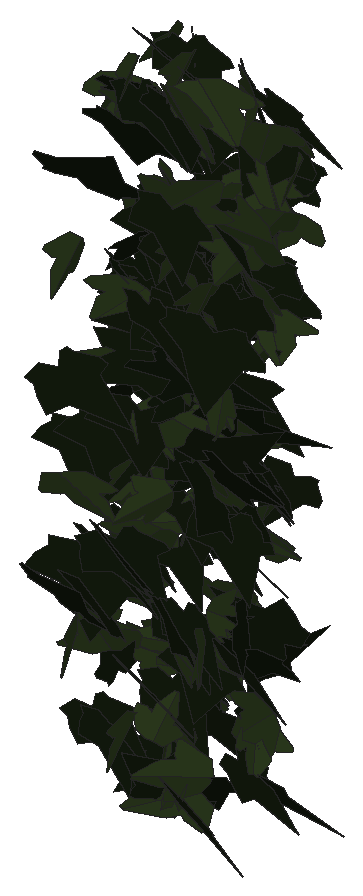
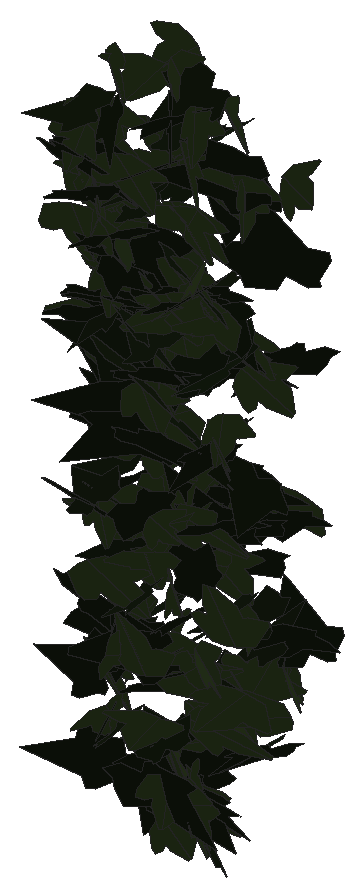
# SketchUp Ruby script. Lengths in millimetres.
U = 1.mm
M = Sketchup.active_model
def pt(a) = Geom::Point3d.new(a.map { |v| v * U })
def face(e, loops, mat)
  f = e.add_face(loops[0].map { |a| pt(a) })
  loops[1..].each { |l| e.add_face(l.map { |a| pt(a) }).erase! }
  f.material = f.back_material = mat if mat
  f
end
# faces: each face lists its corners as indices into pts; further lists are holes
def faces(e, pts, list, mat = nil) = list.each { |f| face(e, (f[0].is_a?(Array) ? f : [f]).map { |l| l.map { |i| pts[i] } }, mat) }
# xy, xz, yz: faces in a plane at the given z, y or x. An outline is a flat list of corners, or four numbers for a rectangle; further outlines are holes
def ring(l) = l.size == 4 ? [[l[0], l[1]], [l[2], l[1]], [l[2], l[3]], [l[0], l[3]]] : l.each_slice(2).to_a
def flat(e, list, mat, &to3) = list.each { |f| face(e, (f[0].is_a?(Array) ? f : [f]).map { |l| ring(l).map { |u, v| to3.(u, v) } }, mat) }
def xy(e, z, list, mat = nil) = flat(e, list, mat) { |x, y| [x, y, z] }
def xz(e, y, list, mat = nil) = flat(e, list, mat) { |x, z| [x, y, z] }
def yz(e, x, list, mat = nil) = flat(e, list, mat) { |y, z| [x, y, z] }
def lines(e, pts, list) = list.each { |a, b| e.add_line(pt(pts[a]), pt(pts[b])) }
# prism: a flat outline (further loops are holes) pulled along v
def prism(e, loops, v, mat = nil)
  f = face(e, loops, mat); d = Geom::Vector3d.new(v.map { |x| x * U })
  f.pushpull(f.normal.samedirection?(d) ? d.length : -d.length)
end
def box(e, o, s, mat = nil) = prism(e, [[o, [o[0] + s[0], o[1], o[2]], [o[0] + s[0], o[1] + s[1], o[2]], [o[0], o[1] + s[1], o[2]]]], [0, 0, s[2]], mat)
def at(x, y, z, deg = 0) = Geom::Transformation.translation(pt([x, y, z])) * Geom::Transformation.rotation(ORIGIN, Z_AXIS, deg.degrees)
def axes(o, x, y, z) = Geom::Transformation.new([*x, 0, *y, 0, *z, 0, *pt(o).to_a, 1])
def part(name) = M.definitions.add(name)
# library, detail: a bought-in or finely detailed component or shape, given as its bounding box
def library(name, o, s) = part(name).tap { |d| box(d.entities, o, s) }
def detail(e, o, s) = box(e.add_group.entities, o, s)
def put(e, d, t, mat = nil) = e.add_instance(d, t).tap { |i| i.material = mat if mat }
def group(e, t, mat = nil) = e.add_group.tap { |g| g.transformation = t; g.material = mat if mat }.entities
root = M.entities
M.materials.add("efeu1").color = [18, 25, 13]
M.materials.add("efeu2").color = [43, 57, 29]
c1 = part("ivyleaf_10")
p = [[0,12.8,-0.8],[-1.5,51.3,-10.9],[-4.9,51,-11.6],[-13.6,26.5,-7.3],[-13.2,15.9,-4.6],[-21.1,19.3,-7.2],
  [-29.5,16.3,-8.3],[-29.2,8.3,-6.2],[-19.7,-9.8,0.5],[-7.6,-13,4],[1,-12.2,5.8],[-0.4,51.1,-11.1],
  [-1.5,51.1,-10.9],[1,-12.4,5.9],[16.9,-12.4,3.5],[35.1,9.1,-5.1],[35,12.9,-6.1],[20.5,16.4,-4.9],
  [15.8,15,-3.8],[15.3,27.6,-7.1],[12.8,31.3,-7.8]]
faces(c1.entities,p,[[0,1,2,3,4,5,6,7,8,9,10],[11,12,0,13,14,15,16,17,18,19,20]],"efeu2")
c2 = part("ivyleaf_9")
p = [[39.1,54.8,31.7],[34.5,51.8,30.2],[-5.3,25.2,17.3],[-17.9,28.3,20.9],[-21.6,21.7,17],[-20.2,4.3,5.3],
  [-22.9,-0.3,2.5],[-17.1,-4,-0.6],[-2,-2.1,-1.2],[-0.7,-15.4,-10.1],[16.6,-22.3,-16.7],[21.1,-15.1,-12.5],
  [32.7,-10.7,-11],[46.1,-1.8,-6.6],[30.8,11.2,3.8]]
faces(c2.entities,p,[[0,1,2,3,4,5,6,7,8,9,10,11,12,13,14]],"efeu1")
put(root,c1,axes([3456.2,839,2506.2],[-0.05855,-0.88523,-0.54951],[0.0878,0.54805,-0.88546],[1.98103,-0.05046,0.023]))
put(root,c2,axes([3449.5,796,2071.7],[-1.0325,-0.74393,-0.21149],[0.2375,0.17075,-0.92073],[1.45265,-0.55668,0.00021]))
put(root,c2,axes([3430.4,804.6,2397.7],[2.21147,0.04712,0.13204],[-0.2513,-0.00281,1.16293],[0.08971,-1.16945,0.00252]))
put(root,c2,axes([3458.7,818.3,2121.9],[0.6766,0.85856,0.21497],[0.18074,0.19332,-0.92916],[-1.67473,0.36773,-0.01343]))
put(root,c2,axes([3437.2,751.5,1880],[1.88054,-0.38188,-0.22943],[0.43927,-0.03862,1.05832],[-0.72521,-1.01364,0.04611]))
put(root,c1,axes([3453.5,863.1,1856.2],[-1.35623,-0.42287,-0.54351],[0.92299,0.24712,-0.82811],[0.93049,-0.86148,0.02925]))
put(root,c1,axes([3459,756.6,1842.1],[0.63988,-0.87304,0.59235],[0.57146,-0.51681,-0.93213],[1.92488,0.44365,0.07982]))
put(root,c1,axes([3442.7,808.3,1816.7],[0.3833,0.20067,0.88907],[0.9971,0.71958,-0.28109],[-1.41943,0.55966,0.04263]))
put(root,c1,axes([3454.9,870.4,1948.7],[-1.6766,-0.05765,0.45851],[0.87841,-0.0604,0.87917],[-0.04398,0.99128,0.08024]))
put(root,c1,axes([3462.5,824.9,1937.6],[-0.86012,0.77193,-0.35043],[0.29869,-0.31406,-0.89423],[-1.58554,-0.47792,0.02164]))
put(root,c1,axes([3468.9,865.7,2211.1],[-0.46907,-0.9224,-0.17623],[0.40552,0.12251,-0.93926],[1.74064,-0.27711,0.17133]))
put(root,c2,axes([3465.7,788.7,1914.7],[-1.45807,-0.78868,-0.4173],[0.58902,0.28099,-1.09925],[1.59275,-0.8259,0.0245]))
put(root,c1,axes([3472.9,839.6,2515.5],[1.83356,0.33112,-0.07589],[-0.14572,-0.01067,-1.01862],[-0.62988,0.96633,0.01475]))
put(root,c1,axes([3477.7,870.6,2191.9],[0.87507,-0.85197,0.10793],[0.11024,-0.09138,-0.96809],[1.63072,0.46336,0.00753]))
put(root,c1,axes([3494.8,774.5,1826.3],[-1.42202,-0.55654,-0.45091],[-0.69155,-0.26701,0.93167],[-1.1748,0.83084,-0.00263]))
put(root,c1,axes([3516.5,838.4,1792.9],[0.35058,-0.06106,-0.98342],[-1.79212,0.28364,-0.19399],[0.5521,0.95947,-0.00524]))
put(root,c2,axes([3488.9,774.9,1868.8],[0.69725,-0.96597,0.06594],[0.01798,0.07406,1.03252],[-1.84263,-0.3648,0.03503]))
put(root,c2,axes([3469.3,819.8,2062.1],[-0.18224,-0.78817,-0.51115],[0.22868,0.49931,-0.79241],[1.7732,-0.1454,0.04966]))
put(root,c1,axes([3491.4,875.1,1903.7],[0.32292,-0.8968,0.20543],[0.0188,-0.20711,-0.91228],[1.7509,0.16762,-0.02809]))
put(root,c2,axes([3457.9,801.7,1932.9],[1.04337,-0.90912,0.265],[0.27555,-0.22214,-1.06159],[1.78107,0.56695,0.009]))
put(root,c1,axes([3475.1,731.8,2049.7],[-1.5112,-0.16262,-0.51737],[0.9773,0.06961,-0.80998],[0.332,-0.94515,0.02936]))
put(root,c2,axes([3489.2,857.2,2069.8],[-0.90329,-0.86682,0.00865],[-0.0062,-0.00807,-0.98825],[1.6498,-0.47463,0.00102]))
put(root,c2,axes([3491.9,802.9,2088],[-1.24855,-0.87187,-0.17445],[0.2087,0.1358,-1.0911],[1.67932,-0.6651,0.0059]))
put(root,c2,axes([3472.8,857,2276.8],[0.91607,-0.83711,-0.26429],[-0.13364,0.26373,-0.96322],[1.66534,0.48164,0.06808]))
put(root,c2,axes([3508.8,831.1,2338.5],[-0.24263,0.82066,-0.53662],[0.13394,-0.53208,-0.83044],[-1.86133,-0.14526,0.01019]))
put(root,c2,axes([3474,838.5,1954.3],[0.7987,-0.9137,-0.14989],[-0.12537,0.13469,-1.00546],[1.75773,0.42479,-0.0036]))
put(root,c2,axes([3512.8,769.1,1803],[-0.07831,0.46001,0.83642],[-0.21739,0.82881,-0.46144],[-1.80369,-0.11987,0.0193]))
put(root,c2,axes([3460.9,829.5,2514.2],[1.52393,-0.06343,0.62804],[1.20109,0.10206,-0.7943],[-0.0256,1.01251,0.1194]))
put(root,c1,axes([3532.5,851,2058],[-0.58176,-0.01907,0.86678],[-1.59127,-0.23667,-0.30006],[0.43654,-0.88811,0.06135]))
put(root,c1,axes([3521.7,822.2,2508.4],[-1.63541,-0.30151,0.46438],[-0.83261,-0.15578,-0.91066],[0.64589,-0.96425,0.00191]))
put(root,c1,axes([3511.5,756,2208.1],[-0.54628,-0.83052,0.66541],[-0.24497,-0.65704,-0.87559],[2.01052,-0.30572,0.07411]))
put(root,c2,axes([3503.1,797.4,2494.5],[1.67675,0.28104,-0.58194],[-1.08157,-0.13157,-0.92389],[-0.58564,1.04763,0.04009]))
put(root,c2,axes([3485.5,836.9,2180.7],[0.57796,-0.88911,-0.13461],[-0.06381,0.13079,-0.93948],[1.71025,0.30534,0.01044]))
put(root,c2,axes([3493.2,853.7,2164.4],[0.26174,-0.6209,-0.70327],[-0.29911,0.68549,-0.63594],[1.76024,0.20881,-0.00349]))
put(root,c2,axes([3484.2,765.2,1740.8],[0.36644,-0.78435,-0.58696],[0.15735,0.60906,-0.78677],[1.85782,0.10312,0.18241]))
put(root,c1,axes([3485.2,865.8,2349.9],[-1.45326,0.05736,-0.64789],[1.21601,-0.12087,-0.76373],[-0.23171,-0.99409,0.05548]))
put(root,c1,axes([3518.2,792.1,2281.4],[1.73047,-0.05206,-0.47628],[-0.9044,0.03248,-0.91072],[0.11645,1.02592,0.00467]))
put(root,c1,axes([3515.7,790.8,2046.8],[0.30985,0.53463,-0.77905],[-0.6855,-0.69572,-0.55271],[-1.66246,0.38652,0.0827]))
put(root,c1,axes([3505.6,802.1,2570.4],[0.81968,-0.85807,0.41051],[0.36512,-0.36301,-0.96006],[1.77315,0.47142,0.00792]))
put(root,c1,axes([3527.6,866.9,2463.3],[1.55449,-0.08133,-0.53812],[-1.00136,0.13009,-0.81826],[0.26479,0.96942,0.06467]))
put(root,c2,axes([3493.8,691.5,2219.4],[0.40719,-0.62477,-0.93815],[-0.12391,0.94645,-0.64515],[2.1416,0.17355,0.14105]))
put(root,c1,axes([3515.9,855.8,2588],[-0.24171,-0.95611,-0.36612],[0.2145,0.35363,-0.96258],[1.93667,-0.15849,0.06092]))
put(root,c1,axes([3511.6,863.5,2399.3],[-0.91151,0.85947,-0.04097],[0.08042,-0.02334,-0.98357],[-1.63563,-0.48012,-0.02552]))
put(root,c1,axes([3520.6,852.4,1685],[0.10828,-0.98371,-0.05333],[0.00049,0.05344,-0.98534],[1.87494,0.05679,0.00334]))
put(root,c1,axes([3531.2,863.1,2463],[1.32725,-0.36658,-0.58266],[-0.76445,0.45689,-0.7682],[1.06398,0.78555,0.1749]))
put(root,c2,axes([3500.5,870.9,2376.3],[0.59292,-0.85778,-0.38902],[-0.16466,0.38195,-0.91149],[1.785,0.32016,0.04514]))
put(root,c2,axes([3532.9,814.1,1625.1],[0.03831,0.3719,0.82199],[-0.09802,0.82133,-0.37034],[-1.71428,-0.03865,0.03954]))
put(root,c2,axes([3492.8,828.5,2273],[0.28932,-0.85598,0.74744],[0.53156,-0.70283,-0.86169],[2.09644,0.29633,0.11534]))
put(root,c2,axes([3546.1,838.5,2379.9],[-0.47343,0.83909,0.45306],[-0.41898,0.40504,-0.87103],[-1.76585,-0.32107,0.0852]))
put(root,c2,axes([3506.4,763.9,1726],[0.08951,-0.9871,0.13749],[0.00027,-0.13763,-0.9882],[1.89678,0.0466,-0.00635]))
put(root,c1,axes([3542.6,792.9,1978.4],[-1.01753,-0.74223,0.50533],[-0.58366,-0.40182,-0.91466],[1.60616,-0.61623,-0.01224]))
put(root,c2,axes([3518,805.5,2120.9],[-1.14608,-0.61477,-0.41336],[0.60673,0.26581,-0.85974],[1.2727,-0.68032,0.03762]))
put(root,c1,axes([3543.2,855.4,2383.4],[1.28044,-0.2848,-0.69572],[-1.02944,0.46501,-0.71342],[0.99363,0.84878,0.15741]))
put(root,c2,axes([3498.9,870.2,1999.8],[0.34429,-0.37712,0.89341],[0.6238,-0.83156,-0.41738],[1.737,0.37338,-0.02719]))
put(root,c1,axes([3519.5,816.1,2111.4],[0.21121,0.99056,0.40153],[0.09586,0.3984,-0.99674],[-2.03196,0.12176,-0.00528]))
put(root,c2,axes([3509.9,828.5,2047.3],[-1.03573,0.19753,0.8737],[1.44273,-0.44306,0.57234],[0.90821,0.92909,0.08718]))
put(root,c1,axes([3536.4,847.6,2531.5],[0.87998,-0.78657,-0.53416],[-0.22861,0.54089,-0.90045],[1.79506,0.45448,0.14718]))
put(root,c2,axes([3520.6,810.4,2288.3],[-1.29476,-0.23476,-0.695],[1.34488,0.04481,-0.70683],[0.3749,-0.97152,0.13535]))
put(root,c2,axes([3530.5,846.6,2355.6],[-1.12915,-0.79156,-0.13412],[0.12525,0.11825,-0.98906],[1.52283,-0.59666,-0.0181]))
put(root,c1,axes([3539.6,874.7,1978.1],[-0.50969,0.80978,-0.32486],[-0.4099,-0.39066,-0.79624],[-1.60917,-0.15698,0.30572]))
put(root,c1,axes([3527.3,823.1,2051.4],[0.35266,0.16928,-0.99561],[0.62641,0.94685,0.22224],[1.8171,-0.35926,0.11662]))
put(root,c2,axes([3561.1,766.9,2220.9],[-1.5158,-0.32253,0.45284],[-0.79565,-0.17408,-0.85927],[0.6975,-0.89949,0.00392]))
put(root,c2,axes([3527.6,864.9,2349.5],[-0.49569,-0.94381,-0.16763],[0.05736,0.16556,-0.97897],[1.82346,-0.26177,-0.01477]))
put(root,c2,axes([3523,757.1,1977],[-0.26687,-0.67733,-0.78077],[0.24969,0.76989,-0.69145],[1.95129,-0.19115,-0.0183]))
put(root,c1,axes([3542.7,872.3,1719],[-1.12067,-0.73215,-0.18983],[0.23424,0.14462,-0.93954],[1.42032,-0.60154,0.00517]))
put(root,c2,axes([3559.5,816.2,1677.7],[-1.72308,-0.01366,-0.00853],[0.01624,-0.00012,-0.90546],[0.02599,-0.9054,0.00025]))
put(root,c1,axes([3538.1,655.3,2408.3],[-0.06138,-0.86797,0.78278],[0.50298,-0.76821,-0.84092],[2.16686,0.15373,0.21737]))
put(root,c2,axes([3521.6,800.8,2540.9],[0.54364,-1.0189,-0.20422],[0.00493,0.21249,-1.05655],[1.97774,0.27955,0.05877]))
put(root,c1,axes([3541.6,838.6,1708.9],[0.06023,0.72627,-0.77199],[-0.1642,-0.768,-0.72605],[-2.01054,0.08448,0.03617]))
put(root,c2,axes([3512.5,843.1,2252.2],[0.92438,-0.7106,0.56644],[0.57122,-0.48079,-0.8605],[1.63245,0.57061,-0.01965]))
put(root,c2,axes([3571.7,812.9,2151.3],[-0.7276,0.79811,0.36598],[-0.39908,0.30462,-0.88335],[-1.62269,-0.43279,0.05315]))
put(root,c2,axes([3576.7,874.6,1721.1],[0.40912,0.13655,-1.04401],[-1.73254,-0.51132,-0.25432],[-1.00692,0.93527,0.01339]))
put(root,c2,axes([3533.5,853.7,1935.3],[0.10428,-0.92556,-0.13576],[-0.06246,0.13401,-0.92686],[1.77929,0.05895,-0.02458]))
put(root,c1,axes([3547.2,743.7,1754.2],[0.35848,-0.9537,0.59057],[0.38633,-0.55997,-0.96903],[2.09966,0.26586,0.07747]))
put(root,c2,axes([3564.3,836.8,2466.2],[0.24664,-1.02922,0.25517],[0.04266,0.25967,1.03598],[-2.01765,-0.12032,0.0531]))
put(root,c2,axes([3569.4,838.2,2585.9],[0.25792,0.03149,-1.0264],[-1.66055,0.54947,-0.09834],[1.03058,0.87746,0.09842]))
put(root,c1,axes([3575,824.1,1830.4],[0.07074,0.29167,1.04358],[-0.84482,-0.94845,0.28089],[1.88126,-0.43689,0.0869]))
put(root,c2,axes([3536.5,810.5,2601.9],[1.80901,-0.23897,-0.31139],[-0.47198,0.26675,-0.96171],[0.57905,0.96399,0.18892]))
put(root,c1,axes([3556.5,874.7,2056.3],[-0.46367,-0.63617,0.61967],[0.20683,-0.65909,-0.63391],[1.67751,-0.09458,0.24944]))
put(root,c1,axes([3535.3,864.6,2335.9],[-1.12486,-0.30552,-0.7503],[1.32122,0.28772,-0.66401],[0.79472,-0.91076,0.04193]))
put(root,c1,axes([3565.3,850.1,2167],[1.54095,-0.62266,-0.31627],[-0.48177,0.18963,-1.02139],[1.23876,0.8483,-0.00381]))
put(root,c2,axes([3547.3,840.2,2325.7],[-0.31175,-0.97246,0.28858],[0.00547,-0.29276,-0.98492],[1.93055,-0.1562,0.04939]))
put(root,c1,axes([3531.2,809,1984.3],[0.37953,0.03521,-0.93105],[1.54914,0.45674,0.19161],[0.86289,-0.83547,0.06552]))
put(root,c2,axes([3578.8,808.3,1667.6],[0.38584,0.38091,-0.79878],[-0.74529,-0.69626,-0.43141],[-1.51036,0.44087,0.00882]))
put(root,c1,axes([3557.5,824,2269.3],[-1.93491,-0.16054,0.19002],[0.36093,0.01721,1.02918],[-0.30639,1.03412,0.01237]))
put(root,c2,axes([3572.1,886.9,2253.9],[-1.38699,-0.55795,0.26405],[-0.26271,-0.25088,-0.91111],[1.14504,-0.7334,0.1108]))
put(root,c1,axes([3566.2,842.8,1644.9],[-0.64072,-0.78974,0.45111],[0.06707,-0.49199,-0.835],[1.72966,-0.27347,0.19948]))
put(root,c2,axes([3543.9,859.6,2583.2],[-0.02749,-0.98694,-0.28146],[0.17079,0.27919,-0.9836],[1.94575,-0.03845,0.08236]))
put(root,c2,axes([3546.6,830.2,1768.4],[0.1162,-1.03723,-0.32249],[-0.05097,0.32146,-1.039],[2.06664,0.06625,-0.00749]))
put(root,c2,axes([3579.1,877.7,2164.7],[-1.68894,-0.28168,0.01555],[-0.02912,-0.00322,-0.93105],[0.53612,-0.88755,-0.00156]))
put(root,c2,axes([3536.1,766,1805.7],[1.08873,-0.69663,0.32705],[0.37483,-0.26141,-0.90131],[1.41588,0.60487,-0.01287]))
put(root,c2,axes([3576.7,772.9,1673.3],[0.40564,0.20583,0.91622],[-1.37468,-0.56446,0.29483],[1.1421,-0.75251,0.02946]))
put(root,c1,axes([3575.2,764.9,2049.6],[-0.18675,-0.34448,1.00567],[-0.05657,-1.00866,-0.34841],[2.02238,-0.06002,0.08312]))
put(root,c1,axes([3591.3,790.6,1655.6],[1.38092,0.09793,-0.76954],[-1.45466,-0.08995,-0.7321],[-0.25249,1.05384,0.00903]))
put(root,c2,axes([3548.7,872,1767.7],[-0.01842,-0.61314,0.74194],[0.40637,-0.72486,-0.59624],[1.7862,0.15859,0.1433]))
put(root,c2,axes([3548,888.2,2294.5],[0.24675,-0.87065,0.39052],[0.30422,-0.36873,-0.87512],[1.79041,0.18264,0.09488]))
put(root,c2,axes([3605.7,779.3,2274.4],[-1.54982,0.30247,0.44741],[-0.87225,0.04118,-0.862],[-0.54371,-0.92822,0.10755]))
put(root,c1,axes([3580.9,811.7,1711.4],[0.69048,-1.02114,-0.46893],[-0.30452,0.4408,-1.08367],[2.11677,0.3965,-0.00293]))
put(root,c1,axes([3580.4,869.5,2214.6],[-0.87464,-0.84302,0.16484],[-0.08625,-0.1629,-0.95941],[1.63255,-0.46026,0.03763]))
put(root,c1,axes([3579.4,818.8,2257.9],[-1.75806,-0.38282,0.00582],[-0.01043,-0.00197,-0.99992],[0.7286,-0.92375,-0.00028]))
put(root,c1,axes([3579.6,815.5,2360],[-0.03462,-1.0076,0.41582],[-0.06524,-0.41514,-1.00746],[2.07352,-0.02988,-0.02475]))
put(root,c2,axes([3546.6,727.5,1980.4],[0.09905,-0.53099,0.99543],[0.59177,-0.95115,-0.52363],[2.06403,0.29818,0.10236]))
put(root,c1,axes([3579.6,810.1,2188.5],[-0.12468,0.64096,0.71049],[-0.44617,0.6797,-0.6348],[-1.76564,-0.21702,0.11024]))
put(root,c1,axes([3594.5,824,2070.5],[-1.3866,0.42313,0.49402],[-0.8235,0.23858,-0.84247],[-0.92431,-0.84731,0.00948]))
put(root,c1,axes([3578.2,867.9,2001.4],[1.39691,0.52199,-0.18628],[-0.25719,-0.13124,-0.90023],[-1.02299,0.74579,-0.02804]))
put(root,c1,axes([3574.4,762.1,1746.3],[0.52161,0.65025,-0.65052],[0.48462,0.59861,0.70564],[1.68211,-0.3741,-0.00158]))
put(root,c2,axes([3591.2,868.9,2066.3],[-0.08087,0.29166,-0.91526],[0.23875,-0.90662,-0.29473],[-1.81256,-0.13243,0.00202]))
put(root,c1,axes([3565.2,871.6,1793],[1.39361,0.52314,0.32536],[0.48781,0.20087,-0.89982],[-1.0662,0.77569,0.01359]))
put(root,c1,axes([3574.8,841.9,2004.2],[0.50052,0.95751,0.15924],[0.0911,0.15199,-0.99295],[-1.84511,0.26725,-0.00583]))
put(root,c1,axes([3585.6,801.4,2605.8],[0.08905,-1.00017,0.32262],[0.18587,-0.3174,-0.99816],[1.99144,0.07435,0.07873]))
put(root,c1,axes([3597.2,820.4,2230.6],[-0.7863,0.69461,0.69183],[-0.80629,0.55054,-0.80575],[-1.68262,-0.58841,0.06281]))
put(root,c2,axes([3558.9,828.4,2382.6],[0.32781,0.54015,-0.81604],[0.53642,0.76609,0.56658],[1.78358,-0.32968,-0.02042]))
put(root,c2,axes([3569.1,812.2,1865.8],[0.27717,-1.01866,-0.0126],[-0.00403,0.01243,-1.02901],[1.93885,0.14565,-0.00034]))
put(root,c2,axes([3579.6,872.9,2505.9],[-0.51833,-0.93235,0.29323],[-0.02813,-0.30044,-0.96899],[1.85992,-0.26437,0.06706]))
put(root,c2,axes([3569.2,808.1,2524.9],[-0.20077,-0.86154,0.61105],[0.34852,-0.6197,-0.84213],[1.97978,0.02173,0.21022]))
put(root,c1,axes([3591.7,779.5,1681.3],[1.07895,-0.79841,-0.18709],[-0.15778,0.17048,-0.97873],[1.5527,0.57213,0.03055]))
put(root,c2,axes([3574.4,832.3,2006.8],[-0.42721,-0.89091,0.28966],[0.3361,-0.33276,-0.88662],[1.75099,-0.15349,0.24086]))
put(root,c2,axes([3611.7,860.5,2303.6],[-1.17374,0.77611,-0.04246],[0.06095,-0.02879,-0.99128],[-1.47805,-0.61751,-0.00716]))
put(root,c1,axes([3564.6,811.3,1855.1],[-1.51411,-0.0538,-0.84648],[1.6114,0.01896,-0.79695],[0.09644,-1.16151,0.0262]))
put(root,c2,axes([3574.1,869.6,1962.6],[0.91828,-0.80704,-0.27],[-0.27049,0.2296,-0.94027],[1.5969,0.50297,-0.00401]))
put(root,c2,axes([3571.6,756.1,2299],[0.45298,-0.9804,0.11826],[0.11423,-0.10706,-1.00834],[1.87594,0.24325,0.03284]))
put(root,c1,axes([3580.7,875,1867.5],[-1.5657,0.13145,0.47615],[0.90001,-0.05766,0.83296],[0.27161,0.94878,-0.01535]))
put(root,c2,axes([3613,871.2,2374.2],[-1.63752,0.40877,-0.20405],[0.31882,-0.12253,-0.95181],[-0.80896,-0.87574,0.03792]))
put(root,c1,axes([3616.9,867.3,2497.8],[-1.62017,-0.027,0.49047],[-0.90583,-0.19735,-0.83696],[0.23119,-0.96245,0.15786]))
put(root,c2,axes([3578.9,786.4,2269.7],[-0.14598,-1.02867,-0.49097],[0.1766,0.48481,-1.03026],[2.16212,-0.10905,0.051]))
put(root,c2,axes([3611.1,799.8,2240.4],[0.45278,0.92417,-0.18748],[-0.12675,-0.1764,-0.95409],[-1.79022,0.24623,0.02014]))
put(root,c2,axes([3633.1,857.3,2244.3],[-0.67186,0.84005,0.36834],[-0.60038,0.25941,-0.89396],[-1.63923,-0.43932,0.17645]))
put(root,c2,axes([3601.5,826.7,1814.5],[-0.72046,-0.89782,0.18594],[-0.08994,-0.18179,-0.974],[1.74268,-0.38056,0.02661]))
put(root,c1,axes([3606,830.1,2047.6],[-1.6397,0.40048,-0.04378],[0.07823,-0.01544,-0.95007],[-0.76274,-0.86252,-0.00332]))
put(root,c1,axes([3619,775.4,1697.7],[0.0146,0.20492,1.16685],[-0.37924,-1.15002,0.20328],[2.22261,-0.19757,0.02702]))
put(root,c2,axes([3606.2,788.8,1676.9],[1.25733,0.78429,-0.03153],[-0.05042,-0.01891,-1.02542],[-1.49301,0.66112,0.00808]))
put(root,c1,axes([3627.8,797.1,2146.1],[0.38208,-0.24107,1.13152],[-1.2305,0.92898,0.31263],[-1.82591,-0.67649,0.02609]))
put(root,c1,axes([3615.7,857.3,2398.7],[0.02996,-0.90176,0.44705],[0.05218,-0.44655,-0.90173],[1.91484,0.02628,0.01758]))
put(root,c1,axes([3638.2,880.4,1966.7],[-1.2379,-0.42498,0.68169],[-1.02644,-0.41904,-0.77582],[1.13307,-0.8439,0.04195]))
put(root,c2,axes([3616.9,881.4,2385.7],[-0.58541,0.37254,-0.86401],[0.84392,-0.74434,-0.4788],[-1.5794,-0.53581,0.06441]))
put(root,c1,axes([3615.8,757.4,1860.7],[-0.54256,0.75096,0.54197],[-0.37101,0.5057,-0.80325],[-1.72308,-0.34535,0.0023]))
put(root,c2,axes([3650.1,839.5,2040.4],[-0.6949,0.6723,0.51093],[-1.04611,0.23334,-0.69984],[-1.21999,-0.58302,0.30907]))
put(root,c2,axes([3587.8,841.4,2340.3],[-0.16068,-0.16044,0.99072],[1.90971,0.00694,0.08663],[-0.03925,0.99429,0.15926]))
put(root,c1,axes([3621.7,880.9,1868.1],[0.18384,0.37472,-0.88999],[-0.48078,-0.85347,-0.38677],[-1.77384,0.27016,0.01259]))
put(root,c1,axes([3625.1,834.8,2382.3],[-0.93377,-0.8754,-0.07136],[0.05228,0.0664,-1.00348],[1.67077,-0.49133,-0.00848]))
put(root,c2,axes([3594.1,855,2159.6],[-0.17088,-0.46984,-1.10499],[0.67935,1.04754,-0.47442],[2.18192,-0.36295,0.06117]))
put(root,c2,axes([3584,761,2227],[0.21078,0.16813,-1.16674],[1.1506,0.99792,0.20119],[1.92595,-0.61458,0.0075]))
put(root,c1,axes([3622.2,872.5,2358.2],[-0.74662,-0.87903,-0.171],[0.28838,0.11884,-0.95852],[1.67977,-0.41112,0.08855]))
put(root,c2,axes([3604.1,778.9,1900.1],[0.41332,-1.00721,-0.05802],[-0.01581,0.05756,-1.03035],[1.92004,0.21729,0.004]))
put(root,c1,axes([3601.6,784.6,2143.3],[-0.94418,-0.37935,-0.73161],[1.37353,0.21231,-0.59946],[0.75726,-0.85808,0.17512]))
put(root,c1,axes([3629.6,786.9,2330.7],[-0.21488,-1.04631,0.02761],[0.00062,-0.0278,-1.05238],[1.99203,-0.11286,0.0033]))
put(root,c2,axes([3612.9,750.5,1896.6],[-0.23294,-0.40033,0.93488],[-0.037,-0.94054,-0.4053],[1.93519,-0.06617,0.10479]))
put(root,c1,axes([3593,825.6,2121.6],[-0.26423,-0.24942,-1.05061],[1.83764,0.44555,-0.23337],[0.92005,-0.96153,0.16439]))
put(root,c2,axes([3640.7,855.4,2557.4],[0.47055,0.24996,-0.93266],[-1.65788,0.47307,-0.10414],[0.79277,0.84094,0.33581]))
put(root,c1,axes([3626.6,809.3,1895],[-0.08775,0.53566,0.801],[-0.25321,0.7907,-0.53643],[-1.81637,-0.13611,0.03608]))
put(root,c2,axes([3619.6,886.1,2414.5],[-0.57929,-0.95298,0.01238],[0.03485,-0.01885,-1.00014],[1.81354,-0.30405,0.02318]))
put(root,c1,axes([3613.4,760.1,2447.2],[-1.75121,-0.36627,0.49589],[0.87773,0.18226,0.99036],[-0.77861,1.02925,0.0011]))
put(root,c2,axes([3596.8,829.2,1857.5],[1.29437,0.26796,0.73486],[1.30081,0.26993,-0.73098],[-0.72388,0.96421,0.00042]))
put(root,c2,axes([3632.4,886.2,2329.8],[-1.4893,-0.61482,0.02829],[0.25032,-0.21175,-0.96385],[1.14431,-0.75386,0.24766]))
put(root,c2,axes([3611.2,815.2,2457.2],[1.3397,-0.50862,-0.52755],[-0.31455,0.60247,-0.80138],[1.35874,0.64097,0.33463]))
put(root,c2,axes([3643,876.7,2327.8],[-1.50526,-0.55455,-0.11469],[0.17542,0.06832,-0.96595],[1.06338,-0.79626,-0.003]))
put(root,c1,axes([3648.6,821.2,2442.8],[0.56466,0.72316,-0.64219],[-0.8831,-0.48294,-0.7582],[-1.615,0.51692,0.19006]))
put(root,c1,axes([3624.8,742,2592.1],[-1.3619,0.75391,-0.60071],[0.7729,-0.44273,-1.0394],[-1.66386,-0.82274,0.00887]))
put(root,c1,axes([3626.3,808.6,2190.9],[-0.80007,0.24619,-0.83192],[0.65114,-0.80248,-0.41036],[-1.51737,-0.47417,0.26255]))
put(root,c2,axes([3615,833.4,1983.3],[1.31588,-0.5788,0.15277],[0.22492,-0.09683,-0.90169],[1.11687,0.70143,0.00159]))
put(root,c2,axes([3633,860.7,2309.8],[1.25966,-0.53962,-0.55674],[-0.76556,0.3868,-0.85311],[1.26151,0.77357,0.03821]))
put(root,c2,axes([3635.2,716.8,2462.6],[-0.30455,-1.02549,-0.03512],[-0.00303,0.0358,-1.03788],[1.95286,-0.15987,-0.00709]))
put(root,c1,axes([3627.7,785.8,2584],[1.5707,0.61188,0.42349],[0.64089,0.25685,-1.02737],[-1.26293,0.89133,0.00534]))
put(root,c2,axes([3627.7,843,2242.5],[0.34798,0.92021,-0.39849],[0.14674,0.39095,0.9382],[1.90285,-0.19843,0.00052]))
put(root,c2,axes([3623.9,807.9,2423.6],[0.50373,-0.96173,0.46345],[0.25937,-0.44313,-0.9974],[2.01517,0.29744,0.01253]))
put(root,c2,axes([3647.3,774.4,2280.8],[-1.21717,-0.98527,-0.24235],[0.25318,0.20257,-1.17464],[1.91439,-0.65323,0.00126]))
put(root,c2,axes([3654.4,853.8,1747.7],[-0.30124,0.0297,0.95286],[-0.61725,-0.90997,-0.02551],[1.70615,-0.32396,0.15901]))
put(root,c2,axes([3624.3,749.4,1675.6],[0.95738,-0.86687,0.5011],[0.42494,-0.44955,-1.00183],[1.85766,0.54959,-0.02908]))
put(root,c2,axes([3663.6,801.7,1896],[0.65184,-0.29062,-1.08098],[-1.52751,0.72423,-0.449],[1.485,0.87253,0.01264]))
put(root,c2,axes([3632.4,853.2,2085.2],[0.68573,-0.90096,0.33872],[0.24386,-0.31356,-0.97033],[1.81558,0.3824,0.0024]))
put(root,c2,axes([3654.2,814,2310],[-1.44145,-0.18548,-0.58185],[1.12106,0.02278,-0.77401],[0.30676,-0.9548,0.09457]))
put(root,c1,axes([3633.8,818.2,2132.8],[-1.17889,0.18058,0.88303],[1.55315,-0.34245,0.64249],[0.72815,1.02282,0.05921]))
put(root,c2,axes([3647.3,823.1,2027.7],[-1.23791,0.07003,-0.87715],[1.66691,-0.05353,-0.65375],[-0.16131,-1.09068,-0.02424]))
put(root,c1,axes([3643.4,874,2414.2],[1.05633,-0.64106,0.48861],[0.92253,-0.20853,-0.8242],[1.22566,0.70944,0.19925]))
put(root,c1,axes([3676.9,805.9,2585.7],[0.34014,-0.33915,-0.98707],[-0.57027,0.94261,-0.37813],[1.90277,0.34313,0.06312]))
put(root,c1,axes([3671.9,801.6,2389.5],[-0.86756,-0.70848,0.50873],[-0.16414,-0.53459,-0.82177],[1.65185,-0.42522,0.18553]))
put(root,c1,axes([3667.3,842.7,2030.4],[-0.41365,-0.92722,-0.07315],[0.0323,0.07115,-0.95235],[1.76987,-0.218,0.00029]))
put(root,c1,axes([3668.1,845,2435.8],[0.39725,-0.88624,-0.43695],[-0.03695,0.44282,-0.90744],[1.88019,0.19595,0.07449]))
put(root,c2,axes([3663.4,880.8,2455],[-1.01732,-0.8444,0.10638],[0.02884,-0.13504,-0.99579],[1.61951,-0.52802,0.08455]))
put(root,c2,axes([3643.8,878.2,2059.6],[0.15232,-0.70565,0.66439],[0.33461,-0.64502,-0.70626],[1.81398,0.17823,0.07449]))
put(root,c2,axes([3638.4,813.9,1850.9],[1.06837,-0.8755,0.09688],[0.10303,-0.08038,-1.04001],[1.67325,0.56395,0.00218]))
put(root,c2,axes([3670.5,807.8,1862.7],[1.28915,0.38931,-0.48773],[-0.8601,-0.19038,-0.7796],[-0.81905,0.81268,0.05101]))
put(root,c1,axes([3657.2,773.6,2205.9],[1.35158,-0.58761,0.30462],[0.44356,-0.19618,-0.92174],[1.17901,0.74742,-0.00244]))
put(root,c2,axes([3659.1,875.2,2300.4],[-0.85377,-0.83389,-0.21901],[0.30635,0.16153,-0.94476],[1.61203,-0.47235,0.06355]))
put(root,c2,axes([3674.1,860.9,2501.5],[-1.6024,-0.49876,-0.15488],[0.26417,0.06956,-0.97853],[0.95821,-0.85325,0.01076]))
put(root,c2,axes([3630.3,799.8,2150.1],[1.49411,0.19406,0.84294],[1.55841,0.20012,-0.80868],[-0.53052,1.13437,-0.00154]))
put(root,c1,axes([3681.5,832.4,2534.3],[-1.49133,-0.66818,0.08016],[-0.13256,-0.04185,-1.02971],[1.27392,-0.78657,-0.01331]))
put(root,c1,axes([3687.4,865.3,2407.9],[-1.76959,-0.1154,0.30767],[-0.51841,-0.24579,-0.91537],[0.34981,-0.94804,0.19987]))
put(root,c1,axes([3669.6,852.5,2251.3],[-0.02113,-0.40165,0.90513],[0.40294,-0.88521,-0.39022],[1.84105,0.18913,0.09579]))
put(root,c2,axes([3708.1,822.3,1882.7],[-0.49431,0.29871,0.94969],[-1.16984,0.72396,-0.39581],[-1.4905,-0.66727,-0.0043]))
put(root,c1,axes([3668.9,824.3,2330.2],[-1.30417,0.6821,-0.13138],[0.17104,-0.09595,-0.96685],[-1.31092,-0.6911,0.00456]))
put(root,c1,axes([3676.6,869.6,2522.9],[-1.47015,0.62242,0.08901],[-0.1239,0.06107,-0.992],[-1.1902,-0.77517,-0.00668]))
put(root,c2,axes([3677,882,2057.3],[-1.54312,-0.24209,-0.34921],[0.76729,-0.20065,-0.79697],[0.25545,-0.8597,0.28434]))
put(root,c1,axes([3684.8,830.3,2452.3],[-0.17715,0.93086,-0.54961],[-0.23904,0.5386,0.93348],[2.04344,0.1437,0.06155]))
put(root,c2,axes([3658.7,852.6,1817.7],[0.25424,-0.11991,1.05032],[1.49442,0.72009,-0.01766],[-1.3471,0.77621,0.17864]))
put(root,c2,axes([3703.5,868.1,2488.9],[-1.84752,0.21539,0.07325],[-0.1418,0.00233,-0.99426],[-0.40912,-0.9735,0.01383]))
put(root,c1,axes([3659.7,835.1,2457.6],[1.51457,0.55612,0.33148],[0.52491,0.184,-0.97084],[-1.11477,0.84221,-0.00678]))
put(root,c1,axes([3675,823.4,1752.2],[0.54027,0.96285,-0.40093],[-0.20224,-0.38666,-1.0038],[-1.97468,0.30303,-0.00689]))
put(root,c2,axes([3669.9,746.5,2091.4],[-0.24366,-0.65853,0.99702],[-0.2611,-0.988,-0.67019],[2.25904,-0.18522,0.03008]))
put(root,c1,axes([3647.7,829.3,2008.2],[0.14523,-0.1076,0.90905],[1.74099,0.04286,-0.07172],[-0.06475,0.91124,0.11071]))
put(root,c2,axes([3666.5,781.6,2040],[-0.13465,-1.18144,-0.0314],[0.00415,0.03133,-1.18355],[2.2493,-0.07078,0.0003]))
put(root,c1,axes([3676.7,842.2,2281.4],[1.21703,0.7254,0.09194],[0.10633,0.07331,-0.96699],[-1.38755,0.64187,0.00654]))
put(root,c2,axes([3663.1,764.3,2129.6],[-0.40431,-0.2107,0.91996],[1.79376,0.00185,0.21807],[-0.09374,0.94417,0.20487]))
put(root,c2,axes([3671.9,795.6,1721.6],[1.01067,-0.81397,-0.44891],[-0.32934,0.42139,-0.96878],[1.73819,0.55313,0.07746]))
put(root,c1,axes([3673.4,718.8,1904.3],[0.13174,-0.1292,1.11038],[1.20074,-0.91388,-0.14567],[1.75631,0.63448,0.0163]))
put(root,c2,axes([3662.8,863,2553.1],[1.0889,-0.80984,0.02263],[0.33172,0.09599,-0.97165],[1.50579,0.56448,0.19769]))
put(root,c2,axes([3660,767.7,2109.2],[0.43966,-0.38457,0.85517],[1.0811,-0.64333,-0.44275],[1.41981,0.60894,0.07232]))
put(root,c1,axes([3706.2,791.1,1798],[1.36921,-0.66194,-0.52085],[-0.62107,0.41243,-0.9749],[1.47785,0.78661,0.07286]))
put(root,c1,axes([3736.8,755.4,2446.7],[-0.73505,0.06365,1.14036],[-2.10965,0.26922,-0.39045],[-0.52386,-1.1735,-0.02772]))
put(root,c1,axes([3709.2,813.3,2439.1],[-0.81555,-0.82164,0.33797],[-0.30639,-0.29721,-0.92666],[1.66288,-0.45773,-0.00498]))
put(root,c2,axes([3717.1,773.4,2114.8],[1.03493,0.13295,-0.79417],[-1.52763,0.16577,-0.52185],[0.12197,0.94812,0.20261]))
put(root,c2,axes([3670.8,823.8,1685.3],[1.39892,-0.38675,0.48989],[0.83978,-0.21331,-0.83045],[0.84015,0.85719,0.01437]))
put(root,c1,axes([3707.4,849.6,2489.6],[0.71997,-0.89853,0.15926],[0.16147,-0.13702,-0.9746],[1.72921,0.3869,0.0247]))
